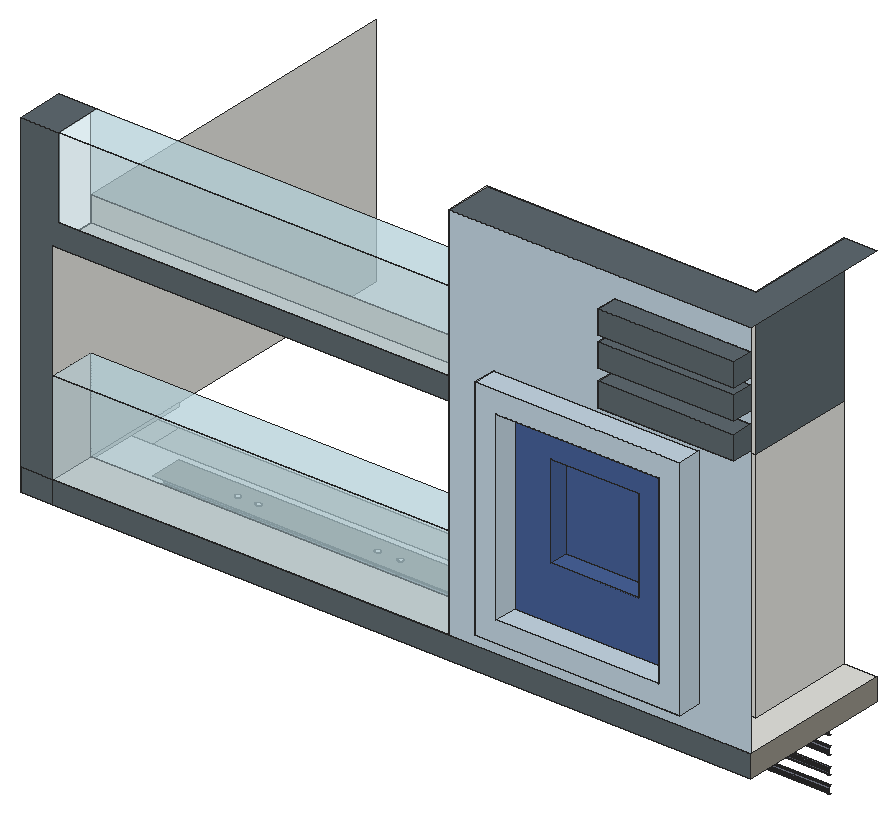
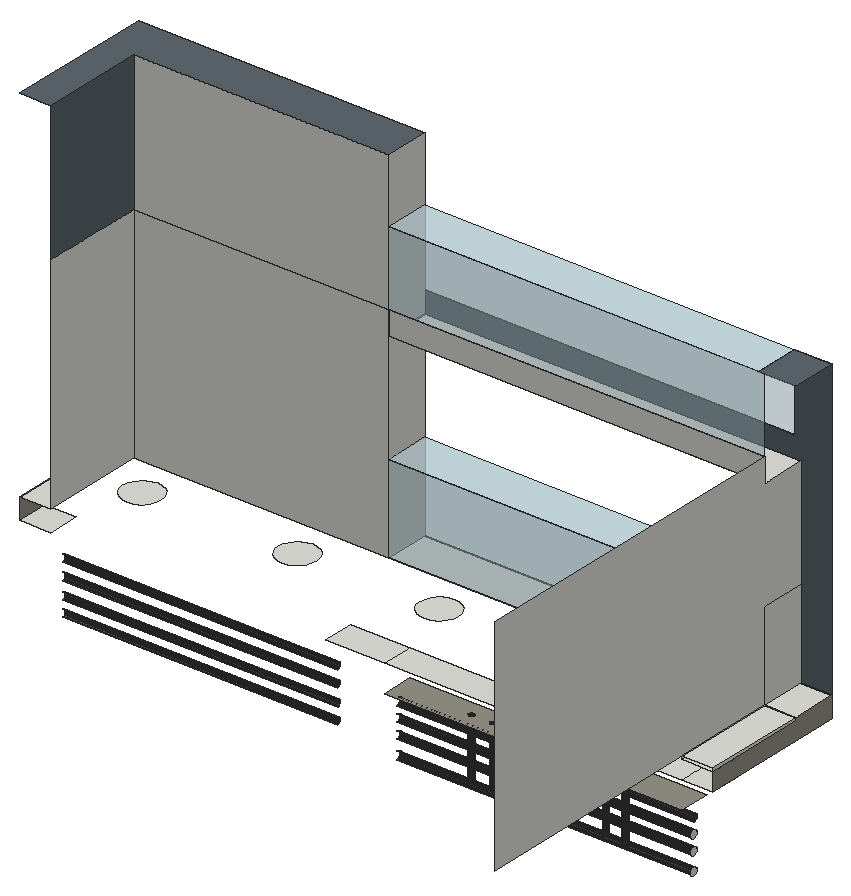
# SketchUp Ruby script. Lengths in inches.
U = 1.inch
M = Sketchup.active_model
def pt(a) = Geom::Point3d.new(a.map { |v| v * U })
def face(e, loops, mat)
  f = e.add_face(loops[0].map { |a| pt(a) })
  loops[1..].each { |l| e.add_face(l.map { |a| pt(a) }).erase! }
  f.material = f.back_material = mat if mat
  f
end
# faces: each face lists its corners as indices into pts; further lists are holes
def faces(e, pts, list, mat = nil) = list.each { |f| face(e, (f[0].is_a?(Array) ? f : [f]).map { |l| l.map { |i| pts[i] } }, mat) }
# xy, xz, yz: faces in a plane at the given z, y or x. An outline is a flat list of corners, or four numbers for a rectangle; further outlines are holes
def ring(l) = l.size == 4 ? [[l[0], l[1]], [l[2], l[1]], [l[2], l[3]], [l[0], l[3]]] : l.each_slice(2).to_a
def flat(e, list, mat, &to3) = list.each { |f| face(e, (f[0].is_a?(Array) ? f : [f]).map { |l| ring(l).map { |u, v| to3.(u, v) } }, mat) }
def xy(e, z, list, mat = nil) = flat(e, list, mat) { |x, y| [x, y, z] }
def xz(e, y, list, mat = nil) = flat(e, list, mat) { |x, z| [x, y, z] }
def yz(e, x, list, mat = nil) = flat(e, list, mat) { |y, z| [x, y, z] }
def lines(e, pts, list) = list.each { |a, b| e.add_line(pt(pts[a]), pt(pts[b])) }
# prism: a flat outline (further loops are holes) pulled along v
def prism(e, loops, v, mat = nil)
  f = face(e, loops, mat); d = Geom::Vector3d.new(v.map { |x| x * U })
  f.pushpull(f.normal.samedirection?(d) ? d.length : -d.length)
end
def box(e, o, s, mat = nil) = prism(e, [[o, [o[0] + s[0], o[1], o[2]], [o[0] + s[0], o[1] + s[1], o[2]], [o[0], o[1] + s[1], o[2]]]], [0, 0, s[2]], mat)
def at(x, y, z, deg = 0) = Geom::Transformation.translation(pt([x, y, z])) * Geom::Transformation.rotation(ORIGIN, Z_AXIS, deg.degrees)
def axes(o, x, y, z) = Geom::Transformation.new([*x, 0, *y, 0, *z, 0, *pt(o).to_a, 1])
def part(name) = M.definitions.add(name)
# library, detail: a bought-in or finely detailed component or shape, given as its bounding box
def library(name, o, s) = part(name).tap { |d| box(d.entities, o, s) }
def detail(e, o, s) = box(e.add_group.entities, o, s)
def put(e, d, t, mat = nil) = e.add_instance(d, t).tap { |i| i.material = mat if mat }
def group(e, t, mat = nil) = e.add_group.tap { |g| g.transformation = t; g.material = mat if mat }.entities
root = M.entities
M.materials.add("[Formica Blue]").color = [71, 97, 152]
M.materials.add("[Formica Graystone]").color = [149, 146, 135]
M.materials.add("[Formica Laminate Dark]").color = [50, 53, 60]
M.materials.add("[Formica Speckled Grey]").color = [94, 105, 111]
M.materials.add("[Metal Steel Textured]").color = [106, 110, 123]
M.materials.add("[Terrazzo Light Blue]").color = [196, 214, 227]
M.materials.add("[Translucent Glass Safety]").color = [204, 235, 244]
M.materials["[Translucent Glass Safety]"].alpha = 0.5
xy(root,48.59,[[[37.72,52.46,82.62,57.16],[68.17,54.44,68.28,54.46,68.39,54.5,68.48,54.57,68.55,54.66,68.59,54.77,68.61,54.88,68.59,54.99,68.55,55.1,68.48,55.19,68.39,55.26,68.28,55.3,68.17,55.32,68.06,55.3,67.95,55.26,67.86,55.19,67.79,55.1,67.75,54.99,67.73,54.88,67.75,54.77,67.79,54.66,67.86,54.57,67.95,54.5,68.06,54.46],[71.42,54.44,71.53,54.46,71.64,54.5,71.73,54.57,71.8,54.66,71.84,54.77,71.86,54.88,71.84,54.99,71.8,55.1,71.73,55.19,71.64,55.26,71.53,55.3,71.42,55.32,71.31,55.3,71.2,55.26,71.11,55.19,71.04,55.1,71,54.99,70.98,54.88,71,54.77,71.04,54.66,71.11,54.57,71.2,54.5,71.31,54.46],[48.11,54.44,48.22,54.46,48.33,54.5,48.42,54.57,48.49,54.66,48.53,54.77,48.54,54.88,48.53,54.99,48.49,55.1,48.42,55.19,48.33,55.26,48.22,55.3,48.11,55.32,47.99,55.3,47.89,55.26,47.8,55.19,47.73,55.1,47.68,54.99,47.67,54.88,47.68,54.77,47.73,54.66,47.8,54.57,47.89,54.5,47.99,54.46],[51.04,54.44,51.16,54.46,51.26,54.5,51.35,54.57,51.42,54.66,51.47,54.77,51.48,54.88,51.47,54.99,51.42,55.1,51.35,55.19,51.26,55.26,51.16,55.3,51.04,55.32,50.93,55.3,50.83,55.26,50.74,55.19,50.67,55.1,50.62,54.99,50.61,54.88,50.62,54.77,50.67,54.66,50.74,54.57,50.83,54.5,50.93,54.46]]],"[Formica Graystone]")
xy(root,52.6875,[[39.58,40.0625,38.83,40.16,38.14,40.45,37.54,40.9,37.09,41.5,36.8,42.19,36.7,42.9375,36.8,43.68,37.09,44.375,37.54,44.97,38.14,45.43,38.83,45.71,39.58,45.8125,40.32,45.71,41.01,45.43,41.61,44.97,42.07,44.375,42.35,43.68,42.45,42.9375,42.35,42.19,42.07,41.5,41.61,40.9,41.01,40.45,40.32,40.16],[63.01,40.0625,62.27,40.16,61.58,40.45,60.98,40.9,60.52,41.5,60.24,42.19,60.14,42.9375,60.24,43.68,60.52,44.375,60.98,44.97,61.58,45.43,62.27,45.71,63.01,45.8125,63.76,45.71,64.45,45.43,65.05,44.97,65.5,44.375,65.79,43.68,65.89,42.9375,65.79,42.19,65.5,41.5,65.05,40.9,64.45,40.45,63.76,40.16],[85.76,40.0625,85.02,40.16,84.33,40.45,83.73,40.9,83.27,41.5,82.99,42.19,82.89,42.9375,82.99,43.68,83.27,44.375,83.73,44.97,84.33,45.43,85.02,45.71,85.76,45.8125,86.51,45.71,87.2,45.43,87.8,44.97,88.25,44.375,88.54,43.68,88.64,42.9375,88.54,42.19,88.25,41.5,87.8,40.9,87.2,40.45,86.51,40.16],[107.2,40.0625,106.46,40.16,105.76,40.45,105.17,40.9,104.71,41.5,104.42,42.19,104.33,42.9375,104.42,43.68,104.71,44.375,105.17,44.97,105.76,45.43,106.46,45.71,107.2,45.8125,107.94,45.71,108.64,45.43,109.23,44.97,109.69,44.375,109.98,43.68,110.08,42.9375,109.98,42.19,109.69,41.5,109.23,40.9,108.64,40.45,107.94,40.16],[130.7,40.0625,129.96,40.16,129.26,40.45,128.67,40.9,128.21,41.5,127.92,42.19,127.83,42.9375,127.92,43.68,128.21,44.375,128.67,44.97,129.26,45.43,129.96,45.71,130.7,45.8125,131.44,45.71,132.14,45.43,132.73,44.97,133.19,44.375,133.48,43.68,133.58,42.9375,133.48,42.19,133.19,41.5,132.73,40.9,132.14,40.45,131.44,40.16],
  [33.03,52.46,37.72,57.16],[37.72,52.46,82.62,57.16],[82.62,52.46,91.56,57.16],[133.09,52.46,137.78,57.16]])
xy(root,55.4375,[[33.03,41.5,37.72,57.16]])
xy(root,55.875,[[33.03,34.66,37.72,41.5],[37.72,34.66,94.51,41.5],[94.51,34.66,94.51,41.5,133.09,41.5,133.09,57.16,137.78,57.16,137.78,34.66],[33.03,41.5,37.72,57.16]])
xy(root,59.6,[[100.88,31.34,130.26,34.66]])
xy(root,62.6,[[103.88,31.34,127.26,34.66]],"[Terrazzo Light Blue]")
xy(root,69.25,[[37.72,34.66,94.51,41.5]],"[Translucent Glass Safety]")
xy(root,70.3,[[109.1,34.66,121.73,37.41]],"[Formica Blue]")
xy(root,83.68,[[109.1,34.66,121.73,37.41]],"[Formica Blue]")
xy(root,85.96,[[37.72,34.66,94.51,41.5]])
xy(root,89.1,[[103.88,31.34,127.26,34.66]],"[Terrazzo Light Blue]")
xy(root,92.1,[[100.88,31.34,130.26,34.66]],"[Terrazzo Light Blue]")
xy(root,94.8125,[[118.28,31.66,137.78,34.66]])
xy(root,98.1875,[[118.28,31.66,137.78,34.66]],"[Formica Speckled Grey]")
xy(root,99.875,[[118.28,31.66,137.78,34.66]])
xy(root,100.8125,[[33.03,34.66,38.52,41.5]],"[Formica Speckled Grey]")
xy(root,100.8125,[[38.52,34.66,94.51,41.5]],"[Translucent Glass Safety]")
xy(root,103.25,[[118.28,31.66,137.78,34.66]],"[Formica Speckled Grey]")
xy(root,104.125,[[118.28,31.66,137.78,34.66]])
xy(root,107.5,[[118.28,31.66,137.78,34.66]],"[Formica Speckled Grey]")
xy(root,110.5625,[[94.51,34.66,137.78,34.66,137.78,57.16,133.09,57.16,133.09,41.5,94.51,41.5]],"[Formica Speckled Grey]")
xz(root,31.34,[[[100.88,59.6,130.26,92.1],[103.88,62.6,127.26,89.1]]],"[Terrazzo Light Blue]")
xz(root,31.66,[[118.28,94.8125,137.78,98.1875],[118.28,99.875,137.78,103.25],[118.28,104.125,137.78,107.5]],"[Formica Speckled Grey]")
xz(root,34.66,[[118.28,94.8125,137.78,98.1875],[118.28,99.875,137.78,103.25],[118.28,104.125,137.78,107.5]])
xz(root,34.66,[[[103.88,62.6,127.26,89.1],[109.1,70.3,121.73,83.68]]],"[Formica Blue]")
xz(root,34.66,[[33.03,52.6875,37.72,55.875],[37.72,52.6875,137.78,55.875],[33.03,55.875,37.72,55.875,37.72,85.96,94.51,85.96,94.51,89.25,38.52,89.25,38.52,100.8125,33.03,100.8125]],"[Formica Speckled Grey]")
xz(root,34.66,[[[94.51,55.875,137.78,55.875,137.78,94.8125,118.28,94.8125,118.28,98.1875,137.78,98.1875,137.78,99.875,118.28,99.875,118.28,103.25,137.78,103.25,137.78,104.125,118.28,104.125,118.28,107.5,137.78,107.5,137.78,110.5625,94.51,110.5625],[100.88,59.6,130.26,92.1]]],"[Terrazzo Light Blue]")
xz(root,34.66,[[37.72,55.875,94.51,69.25],[38.52,89.25,94.51,100.8125]],"[Translucent Glass Safety]")
xz(root,37.41,[[109.1,70.3,121.73,83.68]],"[Formica Blue]")
xz(root,41.5,[[33.03,55.4375,37.72,55.875],[94.51,55.875,133.09,89.5625],[37.72,85.96,94.51,89.5625],[94.51,89.5625,133.09,110.5625]])
xz(root,41.5,[[37.72,55.875,94.51,69.25],[37.72,89.5625,94.51,100.8125]],"[Translucent Glass Safety]")
yz(root,33.03,[[41.5,55.4375,57.16,55.875]])
yz(root,33.03,[[34.66,52.6875,34.66,55.875,41.5,55.875,41.5,55.4375,57.16,55.4375,57.16,52.6875]],"[Formica Graystone]")
yz(root,37.72,[[54.84,38.61,54.69,38.63,54.56,38.68,54.44,38.77,54.35,38.89,54.3,39.03,54.28,39.17,54.3,39.32,54.35,39.45,54.44,39.57,54.56,39.66,54.69,39.72,54.84,39.73,54.99,39.72,55.12,39.66,55.24,39.57,55.33,39.45,55.38,39.32,55.4,39.17,55.38,39.03,55.33,38.89,55.24,38.77,55.12,38.68,54.99,38.63],[54.84,41.36,54.69,41.38,54.56,41.43,54.44,41.52,54.35,41.64,54.3,41.78,54.28,41.92,54.3,42.07,54.35,42.2,54.44,42.32,54.56,42.41,54.69,42.47,54.84,42.48,54.99,42.47,55.12,42.41,55.24,42.32,55.33,42.2,55.38,42.07,55.4,41.92,55.38,41.78,55.33,41.64,55.24,41.52,55.12,41.43,54.99,41.38],[54.84,43.67,54.69,43.69,54.56,43.75,54.44,43.84,54.35,43.95,54.3,44.09,54.28,44.23,54.3,44.38,54.35,44.52,54.44,44.63,54.56,44.72,54.69,44.78,54.84,44.8,54.99,44.78,55.12,44.72,55.24,44.63,55.33,44.52,55.38,44.38,55.4,44.23,55.38,44.09,55.33,43.95,55.24,43.84,55.12,43.75,54.99,43.69],[41.5,55.4375,57.16,55.875],[34.66,55.875,41.5,69.25],
  [41.5,55.875,92.52,55.875,92.52,89.5625,41.5,89.5625,41.5,85.96,34.66,85.96,34.66,69.25,41.5,69.25]])
yz(root,94.51,[[34.66,55.875,41.5,69.25],[34.66,69.25,41.5,85.96],[34.66,85.96,41.5,100.8125],[34.66,100.8125,41.5,110.5625]])
yz(root,100.88,[[31.34,59.6,34.66,92.1]],"[Terrazzo Light Blue]")
yz(root,103.88,[[31.34,62.6,34.66,89.1]],"[Terrazzo Light Blue]")
yz(root,109.1,[[34.66,70.3,37.41,83.68]],"[Formica Blue]")
yz(root,118.28,[[31.66,94.8125,34.66,98.1875],[31.66,99.875,34.66,103.25],[31.66,104.125,34.66,107.5]],"[Formica Speckled Grey]")
yz(root,121.73,[[34.66,70.3,37.41,83.68]],"[Formica Blue]")
yz(root,127.26,[[31.34,62.6,34.66,89.1]],"[Terrazzo Light Blue]")
yz(root,130.26,[[31.34,59.6,34.66,92.1]],"[Terrazzo Light Blue]")
yz(root,133.09,[[41.5,55.875,57.16,89.5625]])
yz(root,133.09,[[41.5,89.5625,57.16,110.5625]],"[Formica Speckled Grey]")
yz(root,137.78,[[34.66,52.6875,57.16,55.875]],"[Formica Graystone]")
yz(root,137.78,[[31.66,94.8125,34.66,98.1875],[31.66,99.875,34.66,103.25],[31.66,104.125,34.66,107.5]],"[Formica Speckled Grey]")
p = [[37.72,54.56,38.68],[37.72,54.69,38.63],[82.62,54.69,38.63],[82.62,54.56,38.68],[37.72,54.84,38.61],[82.62,54.84,38.61],
  [37.72,54.44,38.77],[82.62,54.44,38.77],[37.72,54.35,38.89],[82.62,54.35,38.89],[37.72,54.3,39.03],[82.62,54.3,39.03],
  [37.72,54.28,39.17],[82.62,54.28,39.17],[48.11,54.44,48.59],[47.99,54.46,48.59],[47.99,54.46,38.97],[48.11,54.44,38.97],
  [48.22,54.46,48.59],[48.22,54.46,38.97],[47.89,54.5,48.59],[47.8,54.57,48.59],[47.8,54.57,38.97],[47.89,54.5,38.97],
  [48.33,54.5,48.59],[48.33,54.5,38.97],[48.42,54.57,48.59],[48.42,54.57,38.97],[47.73,54.66,48.59],[47.73,54.66,38.97],
  [48.49,54.66,48.59],[48.49,54.66,38.97],[47.68,54.77,48.59],[47.68,54.77,38.97],[48.53,54.77,48.59],[48.53,54.77,38.97],
  [47.67,54.88,48.59],[47.67,54.88,38.97],[48.54,54.88,48.59],[48.54,54.88,38.97],[37.72,54.3,39.32],[82.62,54.3,39.32],
  [51.04,54.44,48.59],[50.93,54.46,48.59],[50.93,54.46,39.16],[51.04,54.44,39.16],[51.16,54.46,48.59],[51.16,54.46,39.16],
  [50.83,54.5,48.59],[50.74,54.57,48.59],[50.74,54.57,39.16],[50.83,54.5,39.16],[51.26,54.5,48.59],[51.26,54.5,39.16],
  [51.35,54.57,48.59],[51.35,54.57,39.16],[50.67,54.66,48.59],[50.67,54.66,39.16],[51.42,54.66,48.59],[51.42,54.66,39.16],
  [50.62,54.77,48.59],[50.62,54.77,39.16],[51.47,54.77,48.59],[51.47,54.77,39.16],[50.61,54.88,48.59],[50.61,54.88,39.16],
  [51.48,54.88,48.59],[51.48,54.88,39.16],[37.72,54.35,39.45],[82.62,54.35,39.45],[37.72,54.44,39.57],[82.62,54.44,39.57],
  [68.17,54.44,48.59],[68.06,54.46,48.59],[68.06,54.46,39.53],[68.17,54.44,39.53],[68.28,54.46,48.59],[68.28,54.46,39.53],
  [67.95,54.5,48.59],[67.86,54.57,48.59],[67.86,54.57,39.53],[67.95,54.5,39.53],[68.39,54.5,48.59],[68.39,54.5,39.53],
  [68.48,54.57,48.59],[68.48,54.57,39.53],[67.79,54.66,48.59],[67.79,54.66,39.53],[68.55,54.66,48.59],[68.55,54.66,39.53],
  [67.75,54.77,48.59],[67.75,54.77,39.53],[68.59,54.77,48.59],[68.59,54.77,39.53],[67.73,54.88,48.59],[67.73,54.88,39.53],
  [68.61,54.88,48.59],[68.61,54.88,39.53],[37.72,54.56,39.66],[82.62,54.56,39.66],[71.42,54.44,48.59],[71.31,54.46,48.59],
  [71.31,54.46,39.72],[71.42,54.44,39.72],[71.53,54.46,48.59],[71.53,54.46,39.72],[71.2,54.5,48.59],[71.11,54.57,48.59],
  [71.11,54.57,39.72],[71.2,54.5,39.72],[71.64,54.5,48.59],[71.64,54.5,39.72],[71.73,54.57,48.59],[71.73,54.57,39.72],
  [37.72,54.69,39.72],[82.62,54.69,39.72],[71.04,54.66,48.59],[71.04,54.66,39.72],[71.8,54.66,48.59],[71.8,54.66,39.72],
  [37.72,54.84,39.73],[82.62,54.84,39.73],[71,54.77,48.59],[71,54.77,39.72],[71.84,54.77,48.59],[71.84,54.77,39.72],
  [70.98,54.88,48.59],[70.98,54.88,39.72],[71.86,54.88,48.59],[71.86,54.88,39.72],[91.56,54.76,40.26],[91.56,54.9,40.2],
  [133.09,54.9,40.2],[133.09,54.76,40.26],[91.56,54.55,40.46],[91.56,54.64,40.35],[133.09,54.64,40.35],[133.09,54.55,40.46],
  [91.56,54.5,40.6],[133.09,54.5,40.6],[91.56,54.48,40.75],[133.09,54.48,40.75],[91.56,54.5,40.89],[133.09,54.5,40.89],
  [91.56,54.55,41.03],[133.09,54.55,41.03],[91.56,54.64,41.14],[133.09,54.64,41.14],[91.56,54.76,41.23],[133.09,54.76,41.23],
  [91.56,54.9,41.29],[133.09,54.9,41.29],[37.72,54.44,41.52],[37.72,54.56,41.43],[82.62,54.56,41.43],[82.62,54.44,41.52],
  [37.72,54.69,41.38],[82.62,54.69,41.38],[37.72,54.84,41.36],[82.62,54.84,41.36],[37.72,54.35,41.64],[82.62,54.35,41.64],
  [37.72,54.3,41.78],[82.62,54.3,41.78],[37.72,54.28,41.92],[82.62,54.28,41.92],[37.72,54.3,42.07],[82.62,54.3,42.07],
  [37.72,54.35,42.2],[82.62,54.35,42.2],[37.72,54.44,42.32],[82.62,54.44,42.32],[37.72,54.56,42.41],[82.62,54.56,42.41],
  [37.72,54.69,42.47],[82.62,54.69,42.47],[37.72,54.84,42.48],[82.62,54.84,42.48],[91.56,54.64,42.72],[91.56,54.76,42.63],
  [133.09,54.76,42.63],[133.09,54.64,42.72],[91.56,54.9,42.58],[133.09,54.9,42.58],[91.56,54.55,42.84],[133.09,54.55,42.84],
  [91.56,54.5,42.98],[133.09,54.5,42.98],[91.56,54.48,43.12],[133.09,54.48,43.12],[91.56,54.5,43.27],[133.09,54.5,43.27],
  [91.56,54.55,43.4],[133.09,54.55,43.4],[91.56,54.64,43.52],[133.09,54.64,43.52],[91.56,54.76,43.61],[133.09,54.76,43.61],
  [91.56,54.9,43.66],[133.09,54.9,43.66],[37.72,54.44,43.84],[37.72,54.56,43.75],[82.62,54.56,43.75],[82.62,54.44,43.84],
  [37.72,54.69,43.69],[82.62,54.69,43.69],[37.72,54.84,43.67],[82.62,54.84,43.67],[37.72,54.35,43.95],[82.62,54.35,43.95],
  [37.72,54.3,44.09],[82.62,54.3,44.09],[37.72,54.28,44.23],[82.62,54.28,44.23],[37.72,54.3,44.38],[82.62,54.3,44.38],
  [37.72,54.35,44.52],[82.62,54.35,44.52],[37.72,54.44,44.63],[82.62,54.44,44.63],[37.72,54.56,44.72],[82.62,54.56,44.72],
  [37.72,54.69,44.78],[82.62,54.69,44.78],[37.72,54.84,44.8],[82.62,54.84,44.8],[91.56,54.76,45.26],[91.56,54.9,45.2],
  [133.09,54.9,45.2],[133.09,54.76,45.26],[91.56,54.55,45.46],[91.56,54.64,45.35],[133.09,54.64,45.35],[133.09,54.55,45.46],
  [91.56,54.5,45.6],[133.09,54.5,45.6],[91.56,54.48,45.75],[133.09,54.48,45.75],[91.56,54.5,45.89],[133.09,54.5,45.89],
  [91.56,54.55,46.03],[133.09,54.55,46.03],[37.72,54.56,46],[37.72,54.69,45.94],[82.62,54.69,45.94],[82.62,54.56,46],
  [37.72,54.84,45.92],[82.62,54.84,45.92],[37.72,54.44,46.09],[82.62,54.44,46.09],[91.56,54.64,46.14],[133.09,54.64,46.14],
  [37.72,54.35,46.2],[82.62,54.35,46.2],[91.56,54.76,46.23],[133.09,54.76,46.23],[37.72,54.3,46.34],[82.62,54.3,46.34],
  [91.56,54.9,46.29],[133.09,54.9,46.29],[37.72,54.28,46.48],[82.62,54.28,46.48],[37.72,54.3,46.63],[82.62,54.3,46.63],
  [37.72,54.35,46.77],[82.62,54.35,46.77],[37.72,54.44,46.88],[82.62,54.44,46.88],[37.72,54.56,46.97],[82.62,54.56,46.97],
  [37.72,54.69,47.03],[82.62,54.69,47.03],[37.72,54.84,47.05],[82.62,54.84,47.05],[91.56,54.76,47.76],[91.56,54.9,47.7],
  [133.09,54.9,47.7],[133.09,54.76,47.76],[91.56,54.55,47.96],[91.56,54.64,47.85],[133.09,54.64,47.85],[133.09,54.55,47.96],
  [91.56,54.5,48.1],[133.09,54.5,48.1],[91.56,54.48,48.25],[133.09,54.48,48.25],[91.56,54.5,48.39],[133.09,54.5,48.39],
  [91.56,54.55,48.53],[133.09,54.55,48.53],[91.56,54.64,48.64],[133.09,54.64,48.64],[91.56,54.76,48.73],[133.09,54.76,48.73],
  [91.56,54.9,48.79],[133.09,54.9,48.79]]
faces(root,p,[[0,1,2,3],[1,4,5,2],[6,0,3,7],[8,6,7,9],[10,8,9,11],[12,10,11,13],[40,12,13,41],[68,40,41,69],
  [70,68,69,71],[98,70,71,99],[114,98,99,115],[120,114,115,121],[130,131,132,133],[134,135,136,137],[135,130,133,136],[138,134,137,139],
  [140,138,139,141],[142,140,141,143],[144,142,143,145],[146,144,145,147],[148,146,147,149],[150,148,149,151],[152,153,154,155],[153,156,157,154],
  [156,158,159,157],[160,152,155,161],[162,160,161,163],[164,162,163,165],[166,164,165,167],[168,166,167,169],[170,168,169,171],[172,170,171,173],
  [174,172,173,175],[176,174,175,177],[178,179,180,181],[179,182,183,180],[184,178,181,185],[186,184,185,187],[188,186,187,189],[190,188,189,191],
  [192,190,191,193],[194,192,193,195],[196,194,195,197],[198,196,197,199],[200,201,202,203],[201,204,205,202],[204,206,207,205],[208,200,203,209],
  [210,208,209,211],[212,210,211,213],[214,212,213,215],[216,214,215,217],[218,216,217,219],[220,218,219,221],[222,220,221,223],[224,222,223,225],
  [226,227,228,229],[230,231,232,233],[231,226,229,232],[234,230,233,235],[236,234,235,237],[238,236,237,239],[240,238,239,241],[242,243,244,245],
  [243,246,247,244],[248,242,245,249],[250,240,241,251],[252,248,249,253],[254,250,251,255],[256,252,253,257],[258,254,255,259],[260,256,257,261],
  [262,260,261,263],[264,262,263,265],[266,264,265,267],[268,266,267,269],[270,268,269,271],[272,270,271,273],[274,275,276,277],[278,279,280,281],
  [279,274,277,280],[282,278,281,283],[284,282,283,285],[286,284,285,287],[288,286,287,289],[290,288,289,291],[292,290,291,293],[294,292,293,295]],"[Metal Steel Textured]")
faces(root,p,[[14,15,16,17],[18,14,17,19],[20,21,22,23],[15,20,23,16],[24,18,19,25],[26,24,25,27],[21,28,29,22],[30,26,27,31],
  [28,32,33,29],[34,30,31,35],[32,36,37,33],[38,34,35,39],[42,43,44,45],[46,42,45,47],[48,49,50,51],[43,48,51,44],
  [52,46,47,53],[54,52,53,55],[49,56,57,50],[58,54,55,59],[56,60,61,57],[62,58,59,63],[60,64,65,61],[66,62,63,67],
  [72,73,74,75],[76,72,75,77],[78,79,80,81],[73,78,81,74],[82,76,77,83],[84,82,83,85],[79,86,87,80],[88,84,85,89],
  [86,90,91,87],[92,88,89,93],[90,94,95,91],[96,92,93,97],[100,101,102,103],[104,100,103,105],[106,107,108,109],[101,106,109,102],
  [110,104,105,111],[112,110,111,113],[107,116,117,108],[118,112,113,119],[116,122,123,117],[124,118,119,125],[122,126,127,123],[128,124,125,129]],"[Formica Laminate Dark]")
